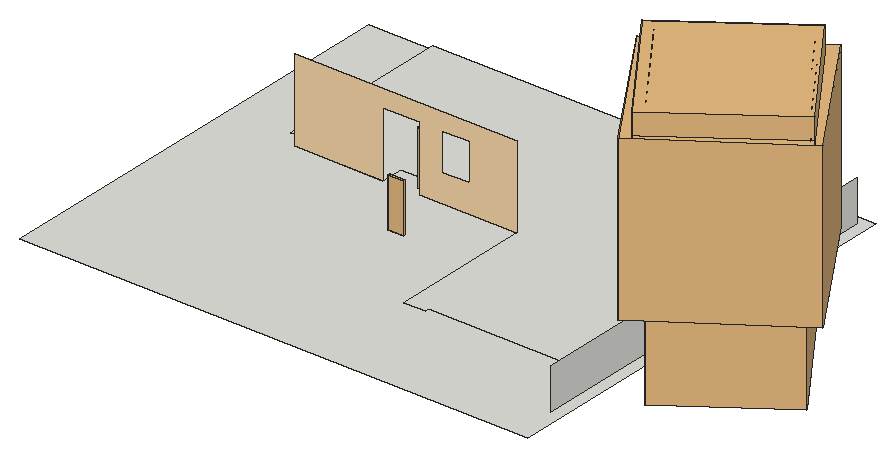
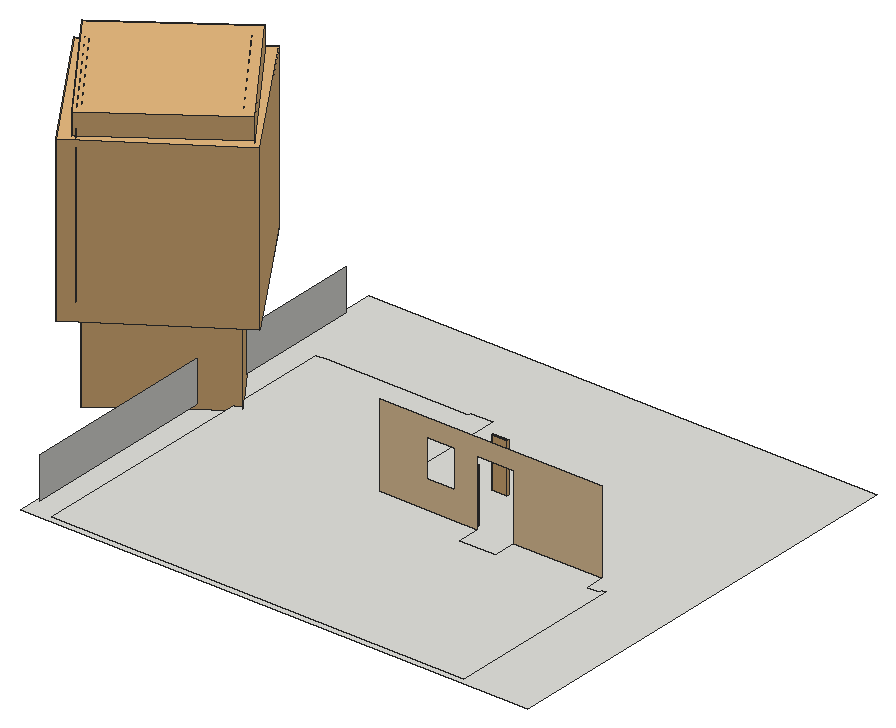
# SketchUp Ruby script. Lengths in inches.
U = 1.inch
M = Sketchup.active_model
def pt(a) = Geom::Point3d.new(a.map { |v| v * U })
def face(e, loops, mat)
  f = e.add_face(loops[0].map { |a| pt(a) })
  loops[1..].each { |l| e.add_face(l.map { |a| pt(a) }).erase! }
  f.material = f.back_material = mat if mat
  f
end
# faces: each face lists its corners as indices into pts; further lists are holes
def faces(e, pts, list, mat = nil) = list.each { |f| face(e, (f[0].is_a?(Array) ? f : [f]).map { |l| l.map { |i| pts[i] } }, mat) }
# xy, xz, yz: faces in a plane at the given z, y or x. An outline is a flat list of corners, or four numbers for a rectangle; further outlines are holes
def ring(l) = l.size == 4 ? [[l[0], l[1]], [l[2], l[1]], [l[2], l[3]], [l[0], l[3]]] : l.each_slice(2).to_a
def flat(e, list, mat, &to3) = list.each { |f| face(e, (f[0].is_a?(Array) ? f : [f]).map { |l| ring(l).map { |u, v| to3.(u, v) } }, mat) }
def xy(e, z, list, mat = nil) = flat(e, list, mat) { |x, y| [x, y, z] }
def xz(e, y, list, mat = nil) = flat(e, list, mat) { |x, z| [x, y, z] }
def yz(e, x, list, mat = nil) = flat(e, list, mat) { |y, z| [x, y, z] }
def lines(e, pts, list) = list.each { |a, b| e.add_line(pt(pts[a]), pt(pts[b])) }
# prism: a flat outline (further loops are holes) pulled along v
def prism(e, loops, v, mat = nil)
  f = face(e, loops, mat); d = Geom::Vector3d.new(v.map { |x| x * U })
  f.pushpull(f.normal.samedirection?(d) ? d.length : -d.length)
end
def box(e, o, s, mat = nil) = prism(e, [[o, [o[0] + s[0], o[1], o[2]], [o[0] + s[0], o[1] + s[1], o[2]], [o[0], o[1] + s[1], o[2]]]], [0, 0, s[2]], mat)
def at(x, y, z, deg = 0) = Geom::Transformation.translation(pt([x, y, z])) * Geom::Transformation.rotation(ORIGIN, Z_AXIS, deg.degrees)
def axes(o, x, y, z) = Geom::Transformation.new([*x, 0, *y, 0, *z, 0, *pt(o).to_a, 1])
def part(name) = M.definitions.add(name)
# library, detail: a bought-in or finely detailed component or shape, given as its bounding box
def library(name, o, s) = part(name).tap { |d| box(d.entities, o, s) }
def detail(e, o, s) = box(e.add_group.entities, o, s)
def put(e, d, t, mat = nil) = e.add_instance(d, t).tap { |i| i.material = mat if mat }
def group(e, t, mat = nil) = e.add_group.tap { |g| g.transformation = t; g.material = mat if mat }.entities
root = M.entities
M.materials.add("028_190k_fullGeometry_Material \#4").color = [120, 148, 64]
M.materials.add("Material \#1").color = [140, 140, 140]
M.materials.add("[0033_NavajoWhite]").color = [255, 222, 173]
c1 = library("3DGeom~9_Defintion",[456.52,-471.89,-18.89],[5.57,1000,5.49])
c2 = library("3DGeom~7_Defintion",[455.56,-471.94,-18.85],[5.55,1000,5.48])
c3 = part("3DGeom~8_Defintion")
xz(c3.entities,-471.94,[[458.125,-17.29,459.53,-16.11,457.73,-17.15],[458.125,-17.29,458.54,-17.29,459.53,-16.11],[458.54,-17.29,458.93,-17.15,459.53,-16.11],[457.73,-17.15,459.53,-16.11,457.42,-16.88],[458.93,-17.15,459.25,-16.88,459.53,-16.11],
  [457.42,-16.88,459.53,-16.11,457.21,-16.52],[459.25,-16.88,459.46,-16.52,459.53,-16.11],[457.21,-16.52,459.53,-16.11,457.14,-16.11],[457.14,-16.11,459.53,-16.11,457.21,-15.7],[459.53,-16.11,457.42,-15.34,457.21,-15.7],
  [459.53,-16.11,457.73,-15.07,457.42,-15.34],[459.53,-16.11,458.125,-14.93,457.73,-15.07],[459.53,-16.11,458.54,-14.93,458.125,-14.93],[459.53,-16.11,458.93,-15.07,458.54,-14.93],[459.53,-16.11,459.25,-15.34,458.93,-15.07],
  [459.53,-16.11,459.46,-15.7,459.25,-15.34]],"Material \#1")
xz(c3.entities,-416.39,[[458.125,-17.29,457.73,-17.15,459.53,-16.11],[458.125,-17.29,459.53,-16.11,458.54,-17.29],[458.54,-17.29,459.53,-16.11,458.93,-17.15],[457.73,-17.15,457.42,-16.88,459.53,-16.11],[458.93,-17.15,459.53,-16.11,459.25,-16.88],
  [457.42,-16.88,457.21,-16.52,459.53,-16.11],[459.25,-16.88,459.53,-16.11,459.46,-16.52],[457.21,-16.52,457.14,-16.11,459.53,-16.11],[457.14,-16.11,457.21,-15.7,459.53,-16.11],[459.53,-16.11,457.21,-15.7,457.42,-15.34],
  [459.53,-16.11,457.42,-15.34,457.73,-15.07],[459.53,-16.11,457.73,-15.07,458.125,-14.93],[459.53,-16.11,458.125,-14.93,458.54,-14.93],[459.53,-16.11,458.54,-14.93,458.93,-15.07],[459.53,-16.11,458.93,-15.07,459.25,-15.34],
  [459.53,-16.11,459.25,-15.34,459.46,-15.7]],"Material \#1")
xz(c3.entities,-27.5,[[458.125,-17.29,459.53,-16.11,457.73,-17.15],[458.125,-17.29,458.54,-17.29,459.53,-16.11],[458.54,-17.29,458.93,-17.15,459.53,-16.11],[457.73,-17.15,459.53,-16.11,457.42,-16.88],[458.93,-17.15,459.25,-16.88,459.53,-16.11],
  [457.42,-16.88,459.53,-16.11,457.21,-16.52],[459.25,-16.88,459.46,-16.52,459.53,-16.11],[457.21,-16.52,459.53,-16.11,457.14,-16.11],[457.14,-16.11,459.53,-16.11,457.21,-15.7],[459.53,-16.11,457.42,-15.34,457.21,-15.7],
  [459.53,-16.11,457.73,-15.07,457.42,-15.34],[459.53,-16.11,458.125,-14.93,457.73,-15.07],[459.53,-16.11,458.54,-14.93,458.125,-14.93],[459.53,-16.11,458.93,-15.07,458.54,-14.93],[459.53,-16.11,459.25,-15.34,458.93,-15.07],
  [459.53,-16.11,459.46,-15.7,459.25,-15.34]],"Material \#1")
xz(c3.entities,28.06,[[458.125,-17.29,457.73,-17.15,459.53,-16.11],[458.125,-17.29,459.53,-16.11,458.54,-17.29],[458.54,-17.29,459.53,-16.11,458.93,-17.15],[457.73,-17.15,457.42,-16.88,459.53,-16.11],[458.93,-17.15,459.53,-16.11,459.25,-16.88],
  [457.42,-16.88,457.21,-16.52,459.53,-16.11],[459.25,-16.88,459.53,-16.11,459.46,-16.52],[457.21,-16.52,457.14,-16.11,459.53,-16.11],[457.14,-16.11,457.21,-15.7,459.53,-16.11],[459.53,-16.11,457.21,-15.7,457.42,-15.34],
  [459.53,-16.11,457.42,-15.34,457.73,-15.07],[459.53,-16.11,457.73,-15.07,458.125,-14.93],[459.53,-16.11,458.125,-14.93,458.54,-14.93],[459.53,-16.11,458.54,-14.93,458.93,-15.07],[459.53,-16.11,458.93,-15.07,459.25,-15.34],
  [459.53,-16.11,459.25,-15.34,459.46,-15.7]],"Material \#1")
xz(c3.entities,472.5,[[458.125,-17.29,459.53,-16.11,457.73,-17.15],[458.125,-17.29,458.54,-17.29,459.53,-16.11],[458.54,-17.29,458.93,-17.15,459.53,-16.11],[457.73,-17.15,459.53,-16.11,457.42,-16.88],[458.93,-17.15,459.25,-16.88,459.53,-16.11],
  [457.42,-16.88,459.53,-16.11,457.21,-16.52],[459.25,-16.88,459.46,-16.52,459.53,-16.11],[457.21,-16.52,459.53,-16.11,457.14,-16.11],[457.14,-16.11,459.53,-16.11,457.21,-15.7],[459.53,-16.11,457.42,-15.34,457.21,-15.7],
  [459.53,-16.11,457.73,-15.07,457.42,-15.34],[459.53,-16.11,458.125,-14.93,457.73,-15.07],[459.53,-16.11,458.54,-14.93,458.125,-14.93],[459.53,-16.11,458.93,-15.07,458.54,-14.93],[459.53,-16.11,459.25,-15.34,458.93,-15.07],
  [459.53,-16.11,459.46,-15.7,459.25,-15.34]],"Material \#1")
xz(c3.entities,528.06,[[458.125,-17.29,457.73,-17.15,459.53,-16.11],[458.125,-17.29,459.53,-16.11,458.54,-17.29],[458.54,-17.29,459.53,-16.11,458.93,-17.15],[457.73,-17.15,457.42,-16.88,459.53,-16.11],[458.93,-17.15,459.53,-16.11,459.25,-16.88],
  [457.42,-16.88,457.21,-16.52,459.53,-16.11],[459.25,-16.88,459.53,-16.11,459.46,-16.52],[457.21,-16.52,457.14,-16.11,459.53,-16.11],[457.14,-16.11,457.21,-15.7,459.53,-16.11],[459.53,-16.11,457.21,-15.7,457.42,-15.34],
  [459.53,-16.11,457.42,-15.34,457.73,-15.07],[459.53,-16.11,457.73,-15.07,458.125,-14.93],[459.53,-16.11,458.125,-14.93,458.54,-14.93],[459.53,-16.11,458.54,-14.93,458.93,-15.07],[459.53,-16.11,458.93,-15.07,459.25,-15.34],
  [459.53,-16.11,459.25,-15.34,459.46,-15.7]],"Material \#1")
c4 = library("028_190k_fullGeometry_0",[-319.99,-281.1,-2.15],[577.33,562.38,1159.36])
c5 = library("028_190k_fullGeometry_1",[-333.4,-281.7,421.48],[600.33,578.53,738.83])
c6 = library("028_190k_fullGeometry_2",[-3584003,-3264710,4041818.25],[6566285.5,6460741.75,7903602.75])
c7 = library("028_190k_fullGeometry_3",[-353.86,-324.57,405.22],[652.24,636.69,781.83])
c8 = part("028_190k_fullGeometry_4")
p = [[125.51,152.8,882.93],[125.36,152.82,883.01],[124.8,155.5625,881.05]]
faces(c8.entities,p,[[0,1,2]],"028_190k_fullGeometry_Material \#4")
c9 = part("028_190k_fullGeometry")
g1 = group(c9.entities,at(0,0,0))
put(g1,c4,axes([0,0,0],[0.18998,-0.26642,0],[0.26642,0.18998,0],[0,0,0.32722]))
put(g1,c5,axes([0,0,0],[0.18998,-0.26642,0],[0.26642,0.18998,0],[0,0,0.32722]))
put(g1,c6,axes([0,0,0],[0.00002,-0.00003,0],[0.00003,0.00002,0],[0,0,0.00003]))
put(g1,c7,axes([0,0,0],[0.18998,-0.26642,0],[0.26642,0.18998,0],[0,0,0.32722]))
put(g1,c8,axes([0,0,0],[0.18998,-0.26642,0],[0.26642,0.18998,0],[0,0,0.32722]))
xy(root,-6,[[1338.625,173.9375,2076.625,807.5]])
xy(root,0,[[1777.8125,322.5,1777.8125,528.0625,1636.42,528.0625,1636.42,560.625,1583.17,560.625,1583.17,528.0625,1454.9375,528.0625,1454.9375,555,1437.22,555,1437.22,549.6875,1431.3125,549.6875,1431.3125,807.5,2031.3125,807.5,2031.3125,327.5,2017.03,327.5,2017.03,327.3125,1809.4375,327.3125,1809.4375,322.5]])
xy(root,6.91,[[1632.125,529.87,1632.04,529.89,1632.06,529.91],[1632.125,529.87,1632.06,529.91,1632.13,529.89],[1632.125,529.87,1632.13,529.89,1632.21,529.87],[1632.21,529.87,1632.13,529.89,1632.21,529.89],[1632.21,529.87,1632.21,529.89,1632.29,529.89],
  [1632.04,529.89,1631.98,529.93,1632,529.94],[1632.04,529.89,1632,529.94,1632.06,529.91],[1632.21,529.89,1632.28,529.91,1632.29,529.89],[1632.29,529.89,1632.28,529.91,1632.36,529.93],[1632.28,529.91,1632.34,529.94,1632.36,529.93],
  [1631.98,529.93,1631.93,529.98,1631.96,529.99],[1631.98,529.93,1631.96,529.99,1632,529.94],[1632.36,529.93,1632.34,529.94,1632.4,529.98],[1632.34,529.94,1632.38,529.99,1632.4,529.98],[1631.93,529.98,1631.92,530.04,1631.94,530.04],
  [1631.93,529.98,1631.94,530.04,1631.96,529.99],[1632.4,529.98,1632.38,529.99,1632.42,530.04],[1632.38,529.99,1632.39,530.04,1632.42,530.04],[1631.92,530.04,1631.93,530.1,1631.96,530.1],[1631.92,530.04,1631.96,530.1,1631.94,530.04],
  [1632.39,530.04,1632.38,530.1,1632.4,530.1],[1632.39,530.04,1632.4,530.1,1632.42,530.04],[1631.93,530.1,1631.98,530.15,1632,530.14],[1631.93,530.1,1632,530.14,1631.96,530.1],[1632.38,530.1,1632.34,530.14,1632.36,530.15],
  [1632.38,530.1,1632.36,530.15,1632.4,530.1],[1632,530.14,1631.98,530.15,1632.06,530.18],[1632.34,530.14,1632.28,530.18,1632.29,530.19],[1632.34,530.14,1632.29,530.19,1632.36,530.15],[1631.98,530.15,1632.04,530.19,1632.06,530.18],
  [1632.06,530.18,1632.04,530.19,1632.13,530.2],[1632.28,530.18,1632.21,530.2,1632.21,530.21],[1632.28,530.18,1632.21,530.21,1632.29,530.19],[1632.04,530.19,1632.125,530.21,1632.13,530.2],[1632.13,530.2,1632.125,530.21,1632.21,530.2],
  [1632.21,530.2,1632.125,530.21,1632.21,530.21]],"Material \#1")
xy(root,6.93,[[1632.125,529.87,1632.13,529.89,1632.04,529.89],[1632.125,529.87,1632.21,529.87,1632.21,529.89],[1632.125,529.87,1632.21,529.89,1632.13,529.89],[1632.21,529.87,1632.28,529.91,1632.21,529.89],[1632.21,529.87,1632.29,529.89,1632.28,529.91],
  [1632.04,529.89,1632.06,529.91,1631.98,529.93],[1632.04,529.89,1632.13,529.89,1632.06,529.91],[1632.29,529.89,1632.34,529.94,1632.28,529.91],[1632.29,529.89,1632.36,529.93,1632.34,529.94],[1632.06,529.91,1632,529.94,1631.98,529.93],
  [1631.98,529.93,1632,529.94,1631.93,529.98],[1632.36,529.93,1632.38,529.99,1632.34,529.94],[1632.36,529.93,1632.4,529.98,1632.38,529.99],[1632,529.94,1631.96,529.99,1631.93,529.98],[1631.93,529.98,1631.96,529.99,1631.92,530.04],
  [1632.4,529.98,1632.39,530.04,1632.38,529.99],[1632.4,529.98,1632.42,530.04,1632.39,530.04],[1631.96,529.99,1631.94,530.04,1631.92,530.04],[1631.92,530.04,1631.94,530.04,1631.93,530.1],[1631.94,530.04,1631.96,530.1,1631.93,530.1],
  [1632.39,530.04,1632.42,530.04,1632.38,530.1],[1632.42,530.04,1632.4,530.1,1632.38,530.1],[1631.93,530.1,1631.96,530.1,1631.98,530.15],[1631.96,530.1,1632,530.14,1631.98,530.15],[1632.38,530.1,1632.4,530.1,1632.34,530.14],
  [1632.4,530.1,1632.36,530.15,1632.34,530.14],[1632,530.14,1632.04,530.19,1631.98,530.15],[1632,530.14,1632.06,530.18,1632.04,530.19],[1632.34,530.14,1632.36,530.15,1632.28,530.18],[1632.36,530.15,1632.29,530.19,1632.28,530.18],
  [1632.06,530.18,1632.125,530.21,1632.04,530.19],[1632.06,530.18,1632.13,530.2,1632.125,530.21],[1632.28,530.18,1632.29,530.19,1632.21,530.2],[1632.29,530.19,1632.21,530.21,1632.21,530.2],[1632.13,530.2,1632.21,530.21,1632.125,530.21],
  [1632.13,530.2,1632.21,530.2,1632.21,530.21]],"Material \#1")
xy(root,10.92,[[1632.125,529.87,1632.04,529.89,1632.13,529.89],[1632.125,529.87,1632.13,529.89,1632.21,529.89],[1632.125,529.87,1632.21,529.89,1632.21,529.87],[1632.21,529.87,1632.21,529.89,1632.28,529.91],[1632.21,529.87,1632.28,529.91,1632.29,529.89],
  [1632.04,529.89,1631.98,529.93,1632.06,529.91],[1632.04,529.89,1632.06,529.91,1632.13,529.89],[1632.29,529.89,1632.28,529.91,1632.34,529.94],[1632.29,529.89,1632.34,529.94,1632.36,529.93],[1632.06,529.91,1631.98,529.93,1632,529.94],
  [1631.98,529.93,1631.93,529.98,1632,529.94],[1632.36,529.93,1632.34,529.94,1632.38,529.99],[1632.36,529.93,1632.38,529.99,1632.4,529.98],[1632,529.94,1631.93,529.98,1631.96,529.99],[1631.93,529.98,1631.92,530.04,1631.96,529.99],
  [1632.4,529.98,1632.38,529.99,1632.39,530.04],[1632.4,529.98,1632.39,530.04,1632.42,530.04],[1631.96,529.99,1631.92,530.04,1631.94,530.04],[1631.92,530.04,1631.93,530.1,1631.94,530.04],[1631.94,530.04,1631.93,530.1,1631.96,530.1],
  [1632.39,530.04,1632.38,530.1,1632.42,530.04],[1632.42,530.04,1632.38,530.1,1632.4,530.1],[1631.93,530.1,1631.98,530.15,1631.96,530.1],[1631.96,530.1,1631.98,530.15,1632,530.14],[1632.38,530.1,1632.34,530.14,1632.4,530.1],
  [1632.4,530.1,1632.34,530.14,1632.36,530.15],[1632,530.14,1631.98,530.15,1632.04,530.19],[1632,530.14,1632.04,530.19,1632.06,530.18],[1632.34,530.14,1632.28,530.18,1632.36,530.15],[1632.36,530.15,1632.28,530.18,1632.29,530.19],
  [1632.06,530.18,1632.04,530.19,1632.125,530.21],[1632.06,530.18,1632.125,530.21,1632.13,530.2],[1632.28,530.18,1632.21,530.2,1632.29,530.19],[1632.29,530.19,1632.21,530.2,1632.21,530.21],[1632.13,530.2,1632.125,530.21,1632.21,530.21],
  [1632.13,530.2,1632.21,530.21,1632.21,530.2]],"Material \#1")
xy(root,10.9375,[[1632.125,529.87,1632.06,529.91,1632.04,529.89],[1632.125,529.87,1632.13,529.89,1632.06,529.91],[1632.125,529.87,1632.21,529.87,1632.13,529.89],[1632.21,529.87,1632.21,529.89,1632.13,529.89],[1632.21,529.87,1632.29,529.89,1632.21,529.89],
  [1632.04,529.89,1632,529.94,1631.98,529.93],[1632.04,529.89,1632.06,529.91,1632,529.94],[1632.21,529.89,1632.29,529.89,1632.28,529.91],[1632.29,529.89,1632.36,529.93,1632.28,529.91],[1632.28,529.91,1632.36,529.93,1632.34,529.94],
  [1631.98,529.93,1631.96,529.99,1631.93,529.98],[1631.98,529.93,1632,529.94,1631.96,529.99],[1632.36,529.93,1632.4,529.98,1632.34,529.94],[1632.34,529.94,1632.4,529.98,1632.38,529.99],[1631.93,529.98,1631.94,530.04,1631.92,530.04],
  [1631.93,529.98,1631.96,529.99,1631.94,530.04],[1632.4,529.98,1632.42,530.04,1632.38,529.99],[1632.38,529.99,1632.42,530.04,1632.39,530.04],[1631.92,530.04,1631.94,530.04,1631.96,530.1],[1631.92,530.04,1631.96,530.1,1631.93,530.1],
  [1632.39,530.04,1632.4,530.1,1632.38,530.1],[1632.39,530.04,1632.42,530.04,1632.4,530.1],[1631.93,530.1,1631.96,530.1,1632,530.14],[1631.93,530.1,1632,530.14,1631.98,530.15],[1632.38,530.1,1632.36,530.15,1632.34,530.14],
  [1632.38,530.1,1632.4,530.1,1632.36,530.15],[1632,530.14,1632.06,530.18,1631.98,530.15],[1632.34,530.14,1632.29,530.19,1632.28,530.18],[1632.34,530.14,1632.36,530.15,1632.29,530.19],[1631.98,530.15,1632.06,530.18,1632.04,530.19],
  [1632.06,530.18,1632.13,530.2,1632.04,530.19],[1632.28,530.18,1632.21,530.21,1632.21,530.2],[1632.28,530.18,1632.29,530.19,1632.21,530.21],[1632.04,530.19,1632.13,530.2,1632.125,530.21],[1632.13,530.2,1632.21,530.2,1632.125,530.21],
  [1632.21,530.2,1632.21,530.21,1632.125,530.21]],"Material \#1")
xz(root,528.0625,[[[1454.9375,0,1583.17,0,1583.17,95.25,1636.42,95.25,1636.42,0,1777.8125,0,1777.8125,120,1454.9375,120],[1668.92,40.75,1708.73,95.25]]],"[0033_NavajoWhite]")
yz(root,2065.5625,[[228.9375,0,786.1875,60]])
put(root,c1,axes([1590.92,531.05,44.51],[0.0898,0,0],[0,0,0.07995],[0,0.06236,0]),"Material \#1")
put(root,c2,axes([1590.92,531.05,44.51],[0.08999,0,0],[0,0,0.08012],[0,0.0625,0]),"Material \#1")
put(root,c3,axes([1590.92,531.05,44.51],[0.08999,0,0],[0,0,0.08012],[0,0.0625,0]),"Material \#1")
g2 = group(root,at(1658.35,443.22,0))
p = [[18.2,0.5,40.71],[17.99,0.52,41.19]]
lines(g2,p,[[0,1]])
detail(g2,[0,0,0],[22.22,2.75,71.73])
put(root,c9,at(2158.9,438.26,-6))
